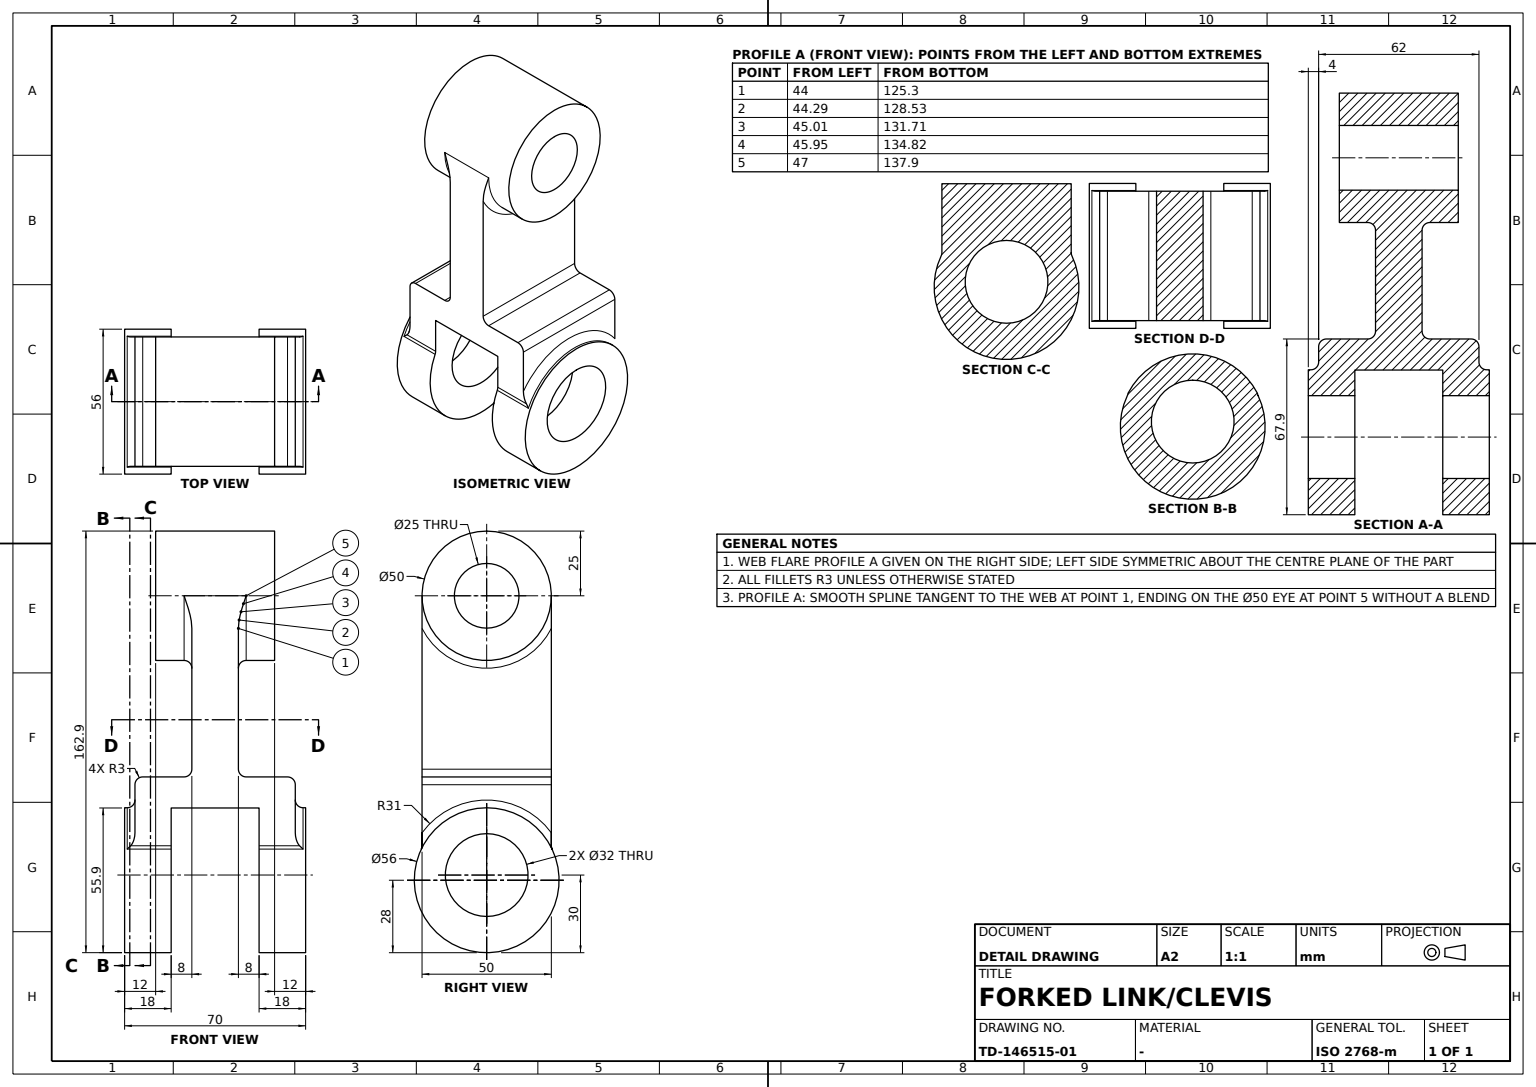
ISO-10303-21;
HEADER;
FILE_DESCRIPTION((''),'2;1');
FILE_NAME('','',(''),(''),'','','');
FILE_SCHEMA(('AUTOMOTIVE_DESIGN'));
ENDSEC;
DATA;
#1=APPLICATION_CONTEXT('');
#2=PRODUCT_CONTEXT('',#1,'mechanical');
#3=PRODUCT('','','',(#2));
#4=PRODUCT_DEFINITION_FORMATION('','',#3);
#5=PRODUCT_DEFINITION_CONTEXT('',#1,'design');
#6=PRODUCT_DEFINITION('','',#4,#5);
#7=PRODUCT_DEFINITION_SHAPE('','',#6);
#8=(LENGTH_UNIT()NAMED_UNIT(*)SI_UNIT(.MILLI.,.METRE.));
#9=(NAMED_UNIT(*)PLANE_ANGLE_UNIT()SI_UNIT($,.RADIAN.));
#10=(NAMED_UNIT(*)SI_UNIT($,.STERADIAN.)SOLID_ANGLE_UNIT());
#11=UNCERTAINTY_MEASURE_WITH_UNIT(LENGTH_MEASURE(0.005),#8,'distance_accuracy_value','');
#12=(GEOMETRIC_REPRESENTATION_CONTEXT(3)GLOBAL_UNCERTAINTY_ASSIGNED_CONTEXT((#11))GLOBAL_UNIT_ASSIGNED_CONTEXT((#8,#9,#10))REPRESENTATION_CONTEXT('',''));
#13=CARTESIAN_POINT('',(-25.,17.,-6.60046));
#14=VERTEX_POINT('',#13);
#15=CARTESIAN_POINT('',(-25.,32.652525,-6.600377));
#16=VERTEX_POINT('',#15);
#17=CARTESIAN_POINT('',(-25.,0.,-6.60046));
#18=DIRECTION('',(0.,-1.,0.));
#19=VECTOR('',#18,1000.);
#20=LINE('',#17,#19);
#21=EDGE_CURVE('',#14,#16,#20,.F.);
#22=ORIENTED_EDGE('',*,*,#21,.F.);
#23=CARTESIAN_POINT('',(-25.,17.,8.));
#24=VERTEX_POINT('',#23);
#25=CARTESIAN_POINT('',(-25.,17.,0.));
#26=DIRECTION('',(0.,0.,-1.));
#27=VECTOR('',#26,1000.);
#28=LINE('',#25,#27);
#29=EDGE_CURVE('',#24,#14,#28,.T.);
#30=ORIENTED_EDGE('',*,*,#29,.F.);
#31=CARTESIAN_POINT('',(-25.,-17.,8.));
#32=VERTEX_POINT('',#31);
#33=CARTESIAN_POINT('',(-25.,0.,8.));
#34=DIRECTION('',(0.,1.,0.));
#35=VECTOR('',#34,1000.);
#36=LINE('',#33,#35);
#37=EDGE_CURVE('',#32,#24,#36,.T.);
#38=ORIENTED_EDGE('',*,*,#37,.F.);
#39=CARTESIAN_POINT('',(-25.,-17.,-6.60046));
#40=VERTEX_POINT('',#39);
#41=CARTESIAN_POINT('',(-25.,-17.,0.));
#42=DIRECTION('',(0.,0.,1.));
#43=VECTOR('',#42,1000.);
#44=LINE('',#41,#43);
#45=EDGE_CURVE('',#40,#32,#44,.T.);
#46=ORIENTED_EDGE('',*,*,#45,.F.);
#47=CARTESIAN_POINT('',(-25.,-32.652602,-6.60046));
#48=VERTEX_POINT('',#47);
#49=EDGE_CURVE('',#40,#48,#20,.T.);
#50=ORIENTED_EDGE('',*,*,#49,.T.);
#51=CARTESIAN_POINT('',(-25.,-31.,-1.574292));
#52=VERTEX_POINT('',#51);
#53=CARTESIAN_POINT('',(-25.,-31.,-2.480429));
#54=CARTESIAN_POINT('',(-25.,-31.277064,-4.242952));
#55=CARTESIAN_POINT('',(-25.,-32.030566,-5.93486));
#56=B_SPLINE_CURVE_WITH_KNOTS('',3,(#51,#53,#54,#55,#47),.UNSPECIFIED.,.F.,.F.,(4,1,4),(0.,0.0026799,0.0053598),.UNSPECIFIED.);
#57=EDGE_CURVE('',#52,#48,#56,.T.);
#58=ORIENTED_EDGE('',*,*,#57,.F.);
#59=CARTESIAN_POINT('',(-25.,-31.,17.));
#60=VERTEX_POINT('',#59);
#61=CARTESIAN_POINT('',(-25.,-31.,0.));
#62=LINE('',#61,#27);
#63=EDGE_CURVE('',#60,#52,#62,.T.);
#64=ORIENTED_EDGE('',*,*,#63,.F.);
#65=CARTESIAN_POINT('',(-25.,-28.,20.));
#66=VERTEX_POINT('',#65);
#67=CARTESIAN_POINT('',(-25.,-28.,17.));
#68=DIRECTION('',(1.,0.,0.));
#69=AXIS2_PLACEMENT_3D('',#67,#68,#26);
#70=CIRCLE('',#69,3.);
#71=EDGE_CURVE('',#66,#60,#70,.T.);
#72=ORIENTED_EDGE('',*,*,#71,.F.);
#73=CARTESIAN_POINT('',(-25.,-12.,20.));
#74=VERTEX_POINT('',#73);
#75=CARTESIAN_POINT('',(-25.,0.,20.));
#76=LINE('',#75,#35);
#77=EDGE_CURVE('',#66,#74,#76,.T.);
#78=ORIENTED_EDGE('',*,*,#77,.T.);
#79=CARTESIAN_POINT('',(-25.,-9.,23.));
#80=VERTEX_POINT('',#79);
#81=CARTESIAN_POINT('',(-25.,-12.,23.));
#82=AXIS2_PLACEMENT_3D('',#81,#68,#26);
#83=CIRCLE('',#82,3.);
#84=EDGE_CURVE('',#74,#80,#83,.T.);
#85=ORIENTED_EDGE('',*,*,#84,.T.);
#86=CARTESIAN_POINT('',(-25.,-9.,77.39048));
#87=VERTEX_POINT('',#86);
#88=CARTESIAN_POINT('',(-25.,-9.,0.));
#89=LINE('',#88,#27);
#90=EDGE_CURVE('',#87,#80,#89,.T.);
#91=ORIENTED_EDGE('',*,*,#90,.F.);
#92=CARTESIAN_POINT('',(-25.,-12.,90.));
#93=VERTEX_POINT('',#92);
#94=CARTESIAN_POINT('',(-25.,-9.,79.576807));
#95=CARTESIAN_POINT('',(-25.,-9.867778,83.829787));
#96=CARTESIAN_POINT('',(-25.,-11.292251,87.956901));
#97=B_SPLINE_CURVE_WITH_KNOTS('',3,(#86,#94,#95,#96,#92),.UNSPECIFIED.,.F.,.F.,(4,1,4),(0.,0.006486638,0.012973277),.UNSPECIFIED.);
#98=EDGE_CURVE('',#87,#93,#97,.T.);
#99=ORIENTED_EDGE('',*,*,#98,.T.);
#100=CARTESIAN_POINT('',(-25.,12.,90.));
#101=VERTEX_POINT('',#100);
#102=CARTESIAN_POINT('',(-25.,0.,90.));
#103=LINE('',#102,#35);
#104=EDGE_CURVE('',#93,#101,#103,.T.);
#105=ORIENTED_EDGE('',*,*,#104,.T.);
#106=CARTESIAN_POINT('',(-25.,9.,77.39048));
#107=VERTEX_POINT('',#106);
#108=CARTESIAN_POINT('',(-25.,9.,79.576807));
#109=CARTESIAN_POINT('',(-25.,9.867778,83.829787));
#110=CARTESIAN_POINT('',(-25.,11.292251,87.956901));
#111=B_SPLINE_CURVE_WITH_KNOTS('',3,(#106,#108,#109,#110,#100),.UNSPECIFIED.,.F.,.F.,(4,1,4),(0.,0.006486638,0.012973277),.UNSPECIFIED.);
#112=EDGE_CURVE('',#107,#101,#111,.T.);
#113=ORIENTED_EDGE('',*,*,#112,.F.);
#114=CARTESIAN_POINT('',(-25.,9.,23.));
#115=VERTEX_POINT('',#114);
#116=CARTESIAN_POINT('',(-25.,9.,0.));
#117=LINE('',#116,#43);
#118=EDGE_CURVE('',#115,#107,#117,.T.);
#119=ORIENTED_EDGE('',*,*,#118,.F.);
#120=CARTESIAN_POINT('',(-25.,12.,20.));
#121=VERTEX_POINT('',#120);
#122=CARTESIAN_POINT('',(-25.,12.,23.));
#123=AXIS2_PLACEMENT_3D('',#122,#68,#26);
#124=CIRCLE('',#123,3.);
#125=EDGE_CURVE('',#115,#121,#124,.T.);
#126=ORIENTED_EDGE('',*,*,#125,.T.);
#127=CARTESIAN_POINT('',(-25.,28.,20.));
#128=VERTEX_POINT('',#127);
#129=EDGE_CURVE('',#121,#128,#76,.T.);
#130=ORIENTED_EDGE('',*,*,#129,.T.);
#131=CARTESIAN_POINT('',(-25.,31.,17.));
#132=VERTEX_POINT('',#131);
#133=CARTESIAN_POINT('',(-25.,28.,17.));
#134=AXIS2_PLACEMENT_3D('',#133,#68,#26);
#135=CIRCLE('',#134,3.);
#136=EDGE_CURVE('',#132,#128,#135,.T.);
#137=ORIENTED_EDGE('',*,*,#136,.F.);
#138=CARTESIAN_POINT('',(-25.,31.,-1.574292));
#139=VERTEX_POINT('',#138);
#140=CARTESIAN_POINT('',(-25.,31.,0.));
#141=LINE('',#140,#43);
#142=EDGE_CURVE('',#139,#132,#141,.T.);
#143=ORIENTED_EDGE('',*,*,#142,.F.);
#144=CARTESIAN_POINT('',(-25.,31.,-2.480411));
#145=CARTESIAN_POINT('',(-25.,31.277053,-4.2429));
#146=CARTESIAN_POINT('',(-25.,32.030524,-5.93477));
#147=B_SPLINE_CURVE_WITH_KNOTS('',3,(#138,#144,#145,#146,#15),.UNSPECIFIED.,.F.,.F.,(4,1,4),(0.,0.002679845,0.005359689),.UNSPECIFIED.);
#148=EDGE_CURVE('',#139,#16,#147,.T.);
#149=ORIENTED_EDGE('',*,*,#148,.T.);
#150=EDGE_LOOP('',(#22,#30,#38,#46,#50,#58,#64,#72,#78,#85,#91,#99,#105,#113,#119,#126,#130,#137,#143,#149));
#151=FACE_BOUND('',#150,.T.);
#152=CARTESIAN_POINT('',(-25.,0.,0.));
#153=AXIS2_PLACEMENT_3D('',#152,#68,#34);
#154=PLANE('',#153);
#155=ADVANCED_FACE('',(#151),#154,.F.);
#156=CARTESIAN_POINT('',(25.,9.,23.));
#157=VERTEX_POINT('',#156);
#158=CARTESIAN_POINT('',(25.,9.,77.39048));
#159=VERTEX_POINT('',#158);
#160=CARTESIAN_POINT('',(25.,9.,0.));
#161=LINE('',#160,#43);
#162=EDGE_CURVE('',#157,#159,#161,.T.);
#163=ORIENTED_EDGE('',*,*,#162,.F.);
#164=CARTESIAN_POINT('',(0.,9.,23.));
#165=VECTOR('',#68,1000.);
#166=LINE('',#164,#165);
#167=EDGE_CURVE('',#115,#157,#166,.T.);
#168=ORIENTED_EDGE('',*,*,#167,.F.);
#169=ORIENTED_EDGE('',*,*,#118,.T.);
#170=CARTESIAN_POINT('',(0.,9.,90.));
#171=AXIS2_PLACEMENT_3D('',#170,#34,#42);
#172=CIRCLE('',#171,28.);
#173=EDGE_CURVE('',#159,#107,#172,.T.);
#174=ORIENTED_EDGE('',*,*,#173,.F.);
#175=EDGE_LOOP('',(#163,#168,#169,#174));
#176=FACE_BOUND('',#175,.T.);
#177=CARTESIAN_POINT('',(0.,9.,20.));
#178=AXIS2_PLACEMENT_3D('',#177,#34,#42);
#179=PLANE('',#178);
#180=ADVANCED_FACE('',(#176),#179,.T.);
#181=CARTESIAN_POINT('',(0.,17.,-33.904594));
#182=VERTEX_POINT('',#181);
#183=CARTESIAN_POINT('',(0.,17.,-17.904594));
#184=AXIS2_PLACEMENT_3D('',#183,#18,#26);
#185=CIRCLE('',#184,16.);
#186=EDGE_CURVE('',#182,#182,#185,.T.);
#187=ORIENTED_EDGE('',*,*,#186,.T.);
#188=EDGE_LOOP('',(#187));
#189=FACE_BOUND('',#188,.T.);
#190=CARTESIAN_POINT('',(0.,35.,-1.904594));
#191=VERTEX_POINT('',#190);
#192=CARTESIAN_POINT('',(0.,35.,-17.904594));
#193=AXIS2_PLACEMENT_3D('',#192,#34,#42);
#194=CIRCLE('',#193,16.);
#195=EDGE_CURVE('',#191,#191,#194,.T.);
#196=ORIENTED_EDGE('',*,*,#195,.T.);
#197=EDGE_LOOP('',(#196));
#198=FACE_BOUND('',#197,.T.);
#199=CARTESIAN_POINT('',(0.,-0.66,-17.904594));
#200=DIRECTION('',(-1.,0.,0.));
#201=AXIS2_PLACEMENT_3D('',#199,#34,#200);
#202=CYLINDRICAL_SURFACE('',#201,16.);
#203=ADVANCED_FACE('',(#189,#198),#202,.F.);
#204=CARTESIAN_POINT('',(-25.290323,34.,-7.887957));
#205=VERTEX_POINT('',#204);
#206=CARTESIAN_POINT('',(25.290323,34.,-7.887957));
#207=VERTEX_POINT('',#206);
#208=CARTESIAN_POINT('',(0.,34.,-19.904594));
#209=AXIS2_PLACEMENT_3D('',#208,#34,#42);
#210=CIRCLE('',#209,28.);
#211=EDGE_CURVE('',#205,#207,#210,.T.);
#212=ORIENTED_EDGE('',*,*,#211,.F.);
#213=CARTESIAN_POINT('',(-25.104442,33.544266,-7.49675));
#214=CARTESIAN_POINT('',(-24.999987,33.086624,-7.064884));
#215=B_SPLINE_CURVE_WITH_KNOTS('',3,(#204,#213,#214,#15),.UNSPECIFIED.,.F.,.F.,(4,4),(-0.000010954,0.001875201),.UNSPECIFIED.);
#216=EDGE_CURVE('',#205,#16,#215,.T.);
#217=ORIENTED_EDGE('',*,*,#216,.T.);
#218=ORIENTED_EDGE('',*,*,#148,.F.);
#219=CARTESIAN_POINT('',(25.,31.,-1.574292));
#220=VERTEX_POINT('',#219);
#221=CARTESIAN_POINT('',(0.,31.,-19.904594));
#222=AXIS2_PLACEMENT_3D('',#221,#34,#42);
#223=CIRCLE('',#222,31.);
#224=EDGE_CURVE('',#139,#220,#223,.T.);
#225=ORIENTED_EDGE('',*,*,#224,.T.);
#226=CARTESIAN_POINT('',(25.,32.652525,-6.600377));
#227=VERTEX_POINT('',#226);
#228=CARTESIAN_POINT('',(25.,31.,-2.480411));
#229=CARTESIAN_POINT('',(25.,31.277053,-4.2429));
#230=CARTESIAN_POINT('',(25.,32.030524,-5.93477));
#231=B_SPLINE_CURVE_WITH_KNOTS('',3,(#219,#228,#229,#230,#226),.UNSPECIFIED.,.F.,.F.,(4,1,4),(0.,0.002679845,0.005359689),.UNSPECIFIED.);
#232=EDGE_CURVE('',#220,#227,#231,.T.);
#233=ORIENTED_EDGE('',*,*,#232,.T.);
#234=CARTESIAN_POINT('',(25.104442,33.544266,-7.49675));
#235=CARTESIAN_POINT('',(24.999987,33.086624,-7.064884));
#236=B_SPLINE_CURVE_WITH_KNOTS('',3,(#206,#234,#235,#226),.UNSPECIFIED.,.F.,.F.,(4,4),(-0.000010954,0.001875201),.UNSPECIFIED.);
#237=EDGE_CURVE('',#207,#227,#236,.T.);
#238=ORIENTED_EDGE('',*,*,#237,.F.);
#239=EDGE_LOOP('',(#212,#217,#218,#225,#233,#238));
#240=FACE_BOUND('',#239,.T.);
#241=DIRECTION('',(-0.613717662,0.,-0.789525574));
#242=AXIS2_PLACEMENT_3D('',#208,#34,#241);
#243=TOROIDAL_SURFACE('',#242,31.,3.);
#244=ADVANCED_FACE('',(#240),#243,.F.);
#245=CARTESIAN_POINT('',(25.,-31.,17.));
#246=VERTEX_POINT('',#245);
#247=CARTESIAN_POINT('',(25.,-31.,-1.574292));
#248=VERTEX_POINT('',#247);
#249=CARTESIAN_POINT('',(25.,-31.,0.));
#250=LINE('',#249,#27);
#251=EDGE_CURVE('',#246,#248,#250,.T.);
#252=ORIENTED_EDGE('',*,*,#251,.F.);
#253=CARTESIAN_POINT('',(0.,-31.,17.));
#254=LINE('',#253,#165);
#255=EDGE_CURVE('',#60,#246,#254,.T.);
#256=ORIENTED_EDGE('',*,*,#255,.F.);
#257=ORIENTED_EDGE('',*,*,#63,.T.);
#258=CARTESIAN_POINT('',(0.,-31.,-19.904594));
#259=AXIS2_PLACEMENT_3D('',#258,#18,#26);
#260=CIRCLE('',#259,31.);
#261=EDGE_CURVE('',#248,#52,#260,.T.);
#262=ORIENTED_EDGE('',*,*,#261,.F.);
#263=EDGE_LOOP('',(#252,#256,#257,#262));
#264=FACE_BOUND('',#263,.T.);
#265=CARTESIAN_POINT('',(0.,-31.,20.));
#266=AXIS2_PLACEMENT_3D('',#265,#18,#26);
#267=PLANE('',#266);
#268=ADVANCED_FACE('',(#264),#267,.T.);
#269=CARTESIAN_POINT('',(0.,23.,102.5));
#270=VERTEX_POINT('',#269);
#271=CARTESIAN_POINT('',(0.,23.,90.));
#272=AXIS2_PLACEMENT_3D('',#271,#34,#42);
#273=CIRCLE('',#272,12.5);
#274=EDGE_CURVE('',#270,#270,#273,.T.);
#275=ORIENTED_EDGE('',*,*,#274,.F.);
#276=EDGE_LOOP('',(#275));
#277=FACE_BOUND('',#276,.T.);
#278=CARTESIAN_POINT('',(0.,23.,115.));
#279=VERTEX_POINT('',#278);
#280=CIRCLE('',#272,25.);
#281=EDGE_CURVE('',#279,#279,#280,.T.);
#282=ORIENTED_EDGE('',*,*,#281,.T.);
#283=EDGE_LOOP('',(#282));
#284=FACE_BOUND('',#283,.T.);
#285=CARTESIAN_POINT('',(0.,23.,0.));
#286=AXIS2_PLACEMENT_3D('',#285,#34,#200);
#287=PLANE('',#286);
#288=ADVANCED_FACE('',(#277,#284),#287,.T.);
#289=CARTESIAN_POINT('',(0.,-35.,-1.904594));
#290=VERTEX_POINT('',#289);
#291=CARTESIAN_POINT('',(0.,-35.,-17.904594));
#292=AXIS2_PLACEMENT_3D('',#291,#34,#42);
#293=CIRCLE('',#292,16.);
#294=EDGE_CURVE('',#290,#290,#293,.T.);
#295=ORIENTED_EDGE('',*,*,#294,.T.);
#296=EDGE_LOOP('',(#295));
#297=FACE_BOUND('',#296,.T.);
#298=CARTESIAN_POINT('',(0.,-35.,8.095406));
#299=VERTEX_POINT('',#298);
#300=CARTESIAN_POINT('',(0.,-35.,-19.904594));
#301=AXIS2_PLACEMENT_3D('',#300,#34,#42);
#302=CIRCLE('',#301,28.);
#303=EDGE_CURVE('',#299,#299,#302,.T.);
#304=ORIENTED_EDGE('',*,*,#303,.F.);
#305=EDGE_LOOP('',(#304));
#306=FACE_BOUND('',#305,.T.);
#307=CARTESIAN_POINT('',(0.,-35.,0.));
#308=AXIS2_PLACEMENT_3D('',#307,#34,#200);
#309=PLANE('',#308);
#310=ADVANCED_FACE('',(#297,#306),#309,.F.);
#311=CARTESIAN_POINT('',(25.,-9.,23.));
#312=VERTEX_POINT('',#311);
#313=CARTESIAN_POINT('',(0.,-9.,23.));
#314=LINE('',#313,#165);
#315=EDGE_CURVE('',#80,#312,#314,.T.);
#316=ORIENTED_EDGE('',*,*,#315,.T.);
#317=CARTESIAN_POINT('',(25.,-9.,77.39048));
#318=VERTEX_POINT('',#317);
#319=CARTESIAN_POINT('',(25.,-9.,0.));
#320=LINE('',#319,#27);
#321=EDGE_CURVE('',#318,#312,#320,.T.);
#322=ORIENTED_EDGE('',*,*,#321,.F.);
#323=CARTESIAN_POINT('',(0.,-9.,90.));
#324=AXIS2_PLACEMENT_3D('',#323,#18,#26);
#325=CIRCLE('',#324,28.);
#326=EDGE_CURVE('',#87,#318,#325,.T.);
#327=ORIENTED_EDGE('',*,*,#326,.F.);
#328=ORIENTED_EDGE('',*,*,#90,.T.);
#329=EDGE_LOOP('',(#316,#322,#327,#328));
#330=FACE_BOUND('',#329,.T.);
#331=PLANE('',#324);
#332=ADVANCED_FACE('',(#330),#331,.T.);
#333=CARTESIAN_POINT('',(0.,-23.,115.));
#334=VERTEX_POINT('',#333);
#335=CARTESIAN_POINT('',(0.,-23.,90.));
#336=AXIS2_PLACEMENT_3D('',#335,#34,#42);
#337=CIRCLE('',#336,25.);
#338=EDGE_CURVE('',#334,#334,#337,.T.);
#339=ORIENTED_EDGE('',*,*,#338,.T.);
#340=EDGE_LOOP('',(#339));
#341=FACE_BOUND('',#340,.T.);
#342=ORIENTED_EDGE('',*,*,#281,.F.);
#343=EDGE_LOOP('',(#342));
#344=FACE_BOUND('',#343,.T.);
#345=CARTESIAN_POINT('',(25.,12.,90.));
#346=VERTEX_POINT('',#345);
#347=CARTESIAN_POINT('',(0.,12.,90.));
#348=AXIS2_PLACEMENT_3D('',#347,#34,#42);
#349=CIRCLE('',#348,25.);
#350=EDGE_CURVE('',#346,#101,#349,.T.);
#351=ORIENTED_EDGE('',*,*,#350,.T.);
#352=ORIENTED_EDGE('',*,*,#104,.F.);
#353=CARTESIAN_POINT('',(25.,-12.,90.));
#354=VERTEX_POINT('',#353);
#355=CARTESIAN_POINT('',(0.,-12.,90.));
#356=AXIS2_PLACEMENT_3D('',#355,#34,#42);
#357=CIRCLE('',#356,25.);
#358=EDGE_CURVE('',#93,#354,#357,.F.);
#359=ORIENTED_EDGE('',*,*,#358,.T.);
#360=CARTESIAN_POINT('',(25.,0.,90.));
#361=LINE('',#360,#35);
#362=EDGE_CURVE('',#354,#346,#361,.T.);
#363=ORIENTED_EDGE('',*,*,#362,.T.);
#364=EDGE_LOOP('',(#351,#352,#359,#363));
#365=FACE_BOUND('',#364,.T.);
#366=CARTESIAN_POINT('',(0.,0.,90.));
#367=AXIS2_PLACEMENT_3D('',#366,#34,#200);
#368=CYLINDRICAL_SURFACE('',#367,25.);
#369=ADVANCED_FACE('',(#341,#344,#365),#368,.T.);
#370=CARTESIAN_POINT('',(25.,-32.652602,-6.60046));
#371=VERTEX_POINT('',#370);
#372=CARTESIAN_POINT('',(25.,-31.,-2.480429));
#373=CARTESIAN_POINT('',(25.,-31.277064,-4.242952));
#374=CARTESIAN_POINT('',(25.,-32.030566,-5.93486));
#375=B_SPLINE_CURVE_WITH_KNOTS('',3,(#247,#372,#373,#374,#370),.UNSPECIFIED.,.F.,.F.,(4,1,4),(0.,0.0026799,0.0053598),.UNSPECIFIED.);
#376=EDGE_CURVE('',#248,#371,#375,.T.);
#377=ORIENTED_EDGE('',*,*,#376,.F.);
#378=ORIENTED_EDGE('',*,*,#261,.T.);
#379=ORIENTED_EDGE('',*,*,#57,.T.);
#380=CARTESIAN_POINT('',(-25.290323,-34.,-7.887957));
#381=VERTEX_POINT('',#380);
#382=CARTESIAN_POINT('',(-25.104453,-33.544293,-7.496773));
#383=CARTESIAN_POINT('',(-25.,-33.086677,-7.064935));
#384=B_SPLINE_CURVE_WITH_KNOTS('',3,(#380,#382,#383,#47),.UNSPECIFIED.,.F.,.F.,(4,4),(-0.000010954,0.00187509),.UNSPECIFIED.);
#385=EDGE_CURVE('',#381,#48,#384,.T.);
#386=ORIENTED_EDGE('',*,*,#385,.F.);
#387=CARTESIAN_POINT('',(25.290323,-34.,-7.887957));
#388=VERTEX_POINT('',#387);
#389=CARTESIAN_POINT('',(0.,-34.,-19.904594));
#390=AXIS2_PLACEMENT_3D('',#389,#34,#42);
#391=CIRCLE('',#390,28.);
#392=EDGE_CURVE('',#388,#381,#391,.F.);
#393=ORIENTED_EDGE('',*,*,#392,.F.);
#394=CARTESIAN_POINT('',(25.104453,-33.544293,-7.496773));
#395=CARTESIAN_POINT('',(25.,-33.086677,-7.064935));
#396=B_SPLINE_CURVE_WITH_KNOTS('',3,(#387,#394,#395,#370),.UNSPECIFIED.,.F.,.F.,(4,4),(-0.000010954,0.00187509),.UNSPECIFIED.);
#397=EDGE_CURVE('',#388,#371,#396,.T.);
#398=ORIENTED_EDGE('',*,*,#397,.T.);
#399=EDGE_LOOP('',(#377,#378,#379,#386,#393,#398));
#400=FACE_BOUND('',#399,.T.);
#401=DIRECTION('',(0.547489236,0.,-0.836812725));
#402=AXIS2_PLACEMENT_3D('',#389,#18,#401);
#403=TOROIDAL_SURFACE('',#402,31.,3.);
#404=ADVANCED_FACE('',(#400),#403,.F.);
#405=CARTESIAN_POINT('',(25.,12.,20.));
#406=VERTEX_POINT('',#405);
#407=CARTESIAN_POINT('',(0.,12.,20.));
#408=LINE('',#407,#165);
#409=EDGE_CURVE('',#121,#406,#408,.T.);
#410=ORIENTED_EDGE('',*,*,#409,.F.);
#411=ORIENTED_EDGE('',*,*,#125,.F.);
#412=ORIENTED_EDGE('',*,*,#167,.T.);
#413=CARTESIAN_POINT('',(25.,12.,23.));
#414=AXIS2_PLACEMENT_3D('',#413,#68,#26);
#415=CIRCLE('',#414,3.);
#416=EDGE_CURVE('',#157,#406,#415,.T.);
#417=ORIENTED_EDGE('',*,*,#416,.T.);
#418=EDGE_LOOP('',(#410,#411,#412,#417));
#419=FACE_BOUND('',#418,.T.);
#420=CARTESIAN_POINT('',(0.,12.,23.));
#421=AXIS2_PLACEMENT_3D('',#420,#68,#18);
#422=CYLINDRICAL_SURFACE('',#421,3.);
#423=ADVANCED_FACE('',(#419),#422,.F.);
#424=ORIENTED_EDGE('',*,*,#294,.F.);
#425=EDGE_LOOP('',(#424));
#426=FACE_BOUND('',#425,.T.);
#427=CARTESIAN_POINT('',(0.,-17.,-1.904594));
#428=VERTEX_POINT('',#427);
#429=CARTESIAN_POINT('',(0.,-17.,-17.904594));
#430=AXIS2_PLACEMENT_3D('',#429,#34,#42);
#431=CIRCLE('',#430,16.);
#432=EDGE_CURVE('',#428,#428,#431,.T.);
#433=ORIENTED_EDGE('',*,*,#432,.T.);
#434=EDGE_LOOP('',(#433));
#435=FACE_BOUND('',#434,.T.);
#436=ADVANCED_FACE('',(#426,#435),#202,.F.);
#437=ORIENTED_EDGE('',*,*,#216,.F.);
#438=CARTESIAN_POINT('',(-25.290323,17.,-7.887957));
#439=VERTEX_POINT('',#438);
#440=CARTESIAN_POINT('',(-25.290323,25.5,-7.887957));
#441=LINE('',#440,#19);
#442=EDGE_CURVE('',#439,#205,#441,.F.);
#443=ORIENTED_EDGE('',*,*,#442,.F.);
#444=CARTESIAN_POINT('',(-28.,17.,-6.60046));
#445=AXIS2_PLACEMENT_3D('',#444,#18,#26);
#446=CIRCLE('',#445,3.);
#447=EDGE_CURVE('',#439,#14,#446,.T.);
#448=ORIENTED_EDGE('',*,*,#447,.T.);
#449=ORIENTED_EDGE('',*,*,#21,.T.);
#450=EDGE_LOOP('',(#437,#443,#448,#449));
#451=FACE_BOUND('',#450,.T.);
#452=CARTESIAN_POINT('',(-28.,0.,-6.60046));
#453=AXIS2_PLACEMENT_3D('',#452,#18,#68);
#454=CYLINDRICAL_SURFACE('',#453,3.);
#455=ADVANCED_FACE('',(#451),#454,.F.);
#456=CARTESIAN_POINT('',(25.,9.,79.576807));
#457=CARTESIAN_POINT('',(25.,9.867778,83.829787));
#458=CARTESIAN_POINT('',(25.,11.292251,87.956901));
#459=B_SPLINE_CURVE_WITH_KNOTS('',3,(#158,#456,#457,#458,#345),.UNSPECIFIED.,.F.,.F.,(4,1,4),(0.,0.006486638,0.012973277),.UNSPECIFIED.);
#460=EDGE_CURVE('',#159,#346,#459,.T.);
#461=ORIENTED_EDGE('',*,*,#460,.F.);
#462=ORIENTED_EDGE('',*,*,#173,.T.);
#463=ORIENTED_EDGE('',*,*,#112,.T.);
#464=ORIENTED_EDGE('',*,*,#350,.F.);
#465=EDGE_LOOP('',(#461,#462,#463,#464));
#466=FACE_BOUND('',#465,.T.);
#467=DIRECTION('',(0.641258302,0.,0.767325087));
#468=AXIS2_PLACEMENT_3D('',#347,#34,#467);
#469=TOROIDAL_SURFACE('',#468,28.,3.);
#470=ADVANCED_FACE('',(#466),#469,.F.);
#471=CARTESIAN_POINT('',(25.,17.,8.));
#472=VERTEX_POINT('',#471);
#473=CARTESIAN_POINT('',(25.,17.,-6.60046));
#474=VERTEX_POINT('',#473);
#475=CARTESIAN_POINT('',(25.,17.,0.));
#476=LINE('',#475,#27);
#477=EDGE_CURVE('',#472,#474,#476,.T.);
#478=ORIENTED_EDGE('',*,*,#477,.T.);
#479=CARTESIAN_POINT('',(25.,0.,-6.60046));
#480=LINE('',#479,#19);
#481=EDGE_CURVE('',#474,#227,#480,.F.);
#482=ORIENTED_EDGE('',*,*,#481,.T.);
#483=ORIENTED_EDGE('',*,*,#232,.F.);
#484=CARTESIAN_POINT('',(25.,31.,17.));
#485=VERTEX_POINT('',#484);
#486=CARTESIAN_POINT('',(25.,31.,0.));
#487=LINE('',#486,#43);
#488=EDGE_CURVE('',#220,#485,#487,.T.);
#489=ORIENTED_EDGE('',*,*,#488,.T.);
#490=CARTESIAN_POINT('',(25.,28.,20.));
#491=VERTEX_POINT('',#490);
#492=CARTESIAN_POINT('',(25.,28.,17.));
#493=AXIS2_PLACEMENT_3D('',#492,#68,#26);
#494=CIRCLE('',#493,3.);
#495=EDGE_CURVE('',#485,#491,#494,.T.);
#496=ORIENTED_EDGE('',*,*,#495,.T.);
#497=CARTESIAN_POINT('',(25.,0.,20.));
#498=LINE('',#497,#35);
#499=EDGE_CURVE('',#406,#491,#498,.T.);
#500=ORIENTED_EDGE('',*,*,#499,.F.);
#501=ORIENTED_EDGE('',*,*,#416,.F.);
#502=ORIENTED_EDGE('',*,*,#162,.T.);
#503=ORIENTED_EDGE('',*,*,#460,.T.);
#504=ORIENTED_EDGE('',*,*,#362,.F.);
#505=CARTESIAN_POINT('',(25.,-9.,79.576807));
#506=CARTESIAN_POINT('',(25.,-9.867778,83.829787));
#507=CARTESIAN_POINT('',(25.,-11.292251,87.956901));
#508=B_SPLINE_CURVE_WITH_KNOTS('',3,(#317,#505,#506,#507,#353),.UNSPECIFIED.,.F.,.F.,(4,1,4),(0.,0.006486638,0.012973277),.UNSPECIFIED.);
#509=EDGE_CURVE('',#318,#354,#508,.T.);
#510=ORIENTED_EDGE('',*,*,#509,.F.);
#511=ORIENTED_EDGE('',*,*,#321,.T.);
#512=CARTESIAN_POINT('',(25.,-12.,20.));
#513=VERTEX_POINT('',#512);
#514=CARTESIAN_POINT('',(25.,-12.,23.));
#515=AXIS2_PLACEMENT_3D('',#514,#68,#26);
#516=CIRCLE('',#515,3.);
#517=EDGE_CURVE('',#513,#312,#516,.T.);
#518=ORIENTED_EDGE('',*,*,#517,.F.);
#519=CARTESIAN_POINT('',(25.,-28.,20.));
#520=VERTEX_POINT('',#519);
#521=EDGE_CURVE('',#520,#513,#498,.T.);
#522=ORIENTED_EDGE('',*,*,#521,.F.);
#523=CARTESIAN_POINT('',(25.,-28.,17.));
#524=AXIS2_PLACEMENT_3D('',#523,#68,#26);
#525=CIRCLE('',#524,3.);
#526=EDGE_CURVE('',#520,#246,#525,.T.);
#527=ORIENTED_EDGE('',*,*,#526,.T.);
#528=ORIENTED_EDGE('',*,*,#251,.T.);
#529=ORIENTED_EDGE('',*,*,#376,.T.);
#530=CARTESIAN_POINT('',(25.,-17.,-6.60046));
#531=VERTEX_POINT('',#530);
#532=EDGE_CURVE('',#531,#371,#480,.T.);
#533=ORIENTED_EDGE('',*,*,#532,.F.);
#534=CARTESIAN_POINT('',(25.,-17.,8.));
#535=VERTEX_POINT('',#534);
#536=CARTESIAN_POINT('',(25.,-17.,0.));
#537=LINE('',#536,#43);
#538=EDGE_CURVE('',#531,#535,#537,.T.);
#539=ORIENTED_EDGE('',*,*,#538,.T.);
#540=CARTESIAN_POINT('',(25.,0.,8.));
#541=LINE('',#540,#35);
#542=EDGE_CURVE('',#535,#472,#541,.T.);
#543=ORIENTED_EDGE('',*,*,#542,.T.);
#544=EDGE_LOOP('',(#478,#482,#483,#489,#496,#500,#501,#502,#503,#504,#510,#511,#518,#522,#527,#528,#529,#533,#539,#543));
#545=FACE_BOUND('',#544,.T.);
#546=CARTESIAN_POINT('',(25.,0.,0.));
#547=AXIS2_PLACEMENT_3D('',#546,#68,#34);
#548=PLANE('',#547);
#549=ADVANCED_FACE('',(#545),#548,.T.);
#550=CARTESIAN_POINT('',(0.,17.,8.));
#551=LINE('',#550,#165);
#552=EDGE_CURVE('',#24,#472,#551,.T.);
#553=ORIENTED_EDGE('',*,*,#552,.T.);
#554=ORIENTED_EDGE('',*,*,#542,.F.);
#555=CARTESIAN_POINT('',(0.,-17.,8.));
#556=LINE('',#555,#165);
#557=EDGE_CURVE('',#32,#535,#556,.T.);
#558=ORIENTED_EDGE('',*,*,#557,.F.);
#559=ORIENTED_EDGE('',*,*,#37,.T.);
#560=EDGE_LOOP('',(#553,#554,#558,#559));
#561=FACE_BOUND('',#560,.T.);
#562=AXIS2_PLACEMENT_3D('',#555,#26,#34);
#563=PLANE('',#562);
#564=ADVANCED_FACE('',(#561),#563,.T.);
#565=ORIENTED_EDGE('',*,*,#481,.F.);
#566=CARTESIAN_POINT('',(25.290323,17.,-7.887957));
#567=VERTEX_POINT('',#566);
#568=CARTESIAN_POINT('',(28.,17.,-6.60046));
#569=AXIS2_PLACEMENT_3D('',#568,#18,#26);
#570=CIRCLE('',#569,3.);
#571=EDGE_CURVE('',#474,#567,#570,.T.);
#572=ORIENTED_EDGE('',*,*,#571,.T.);
#573=CARTESIAN_POINT('',(25.290323,25.5,-7.887957));
#574=LINE('',#573,#35);
#575=EDGE_CURVE('',#567,#207,#574,.T.);
#576=ORIENTED_EDGE('',*,*,#575,.T.);
#577=ORIENTED_EDGE('',*,*,#237,.T.);
#578=EDGE_LOOP('',(#565,#572,#576,#577));
#579=FACE_BOUND('',#578,.T.);
#580=CARTESIAN_POINT('',(28.,0.,-6.60046));
#581=AXIS2_PLACEMENT_3D('',#580,#18,#200);
#582=CYLINDRICAL_SURFACE('',#581,3.);
#583=ADVANCED_FACE('',(#579),#582,.F.);
#584=CARTESIAN_POINT('',(0.,-28.,20.));
#585=LINE('',#584,#165);
#586=EDGE_CURVE('',#66,#520,#585,.T.);
#587=ORIENTED_EDGE('',*,*,#586,.F.);
#588=ORIENTED_EDGE('',*,*,#71,.T.);
#589=ORIENTED_EDGE('',*,*,#255,.T.);
#590=ORIENTED_EDGE('',*,*,#526,.F.);
#591=EDGE_LOOP('',(#587,#588,#589,#590));
#592=FACE_BOUND('',#591,.T.);
#593=CARTESIAN_POINT('',(0.,-28.,17.));
#594=AXIS2_PLACEMENT_3D('',#593,#68,#18);
#595=CYLINDRICAL_SURFACE('',#594,3.);
#596=ADVANCED_FACE('',(#592),#595,.T.);
#597=ORIENTED_EDGE('',*,*,#274,.T.);
#598=EDGE_LOOP('',(#597));
#599=FACE_BOUND('',#598,.T.);
#600=CARTESIAN_POINT('',(0.,-23.,102.5));
#601=VERTEX_POINT('',#600);
#602=CIRCLE('',#336,12.5);
#603=EDGE_CURVE('',#601,#601,#602,.T.);
#604=ORIENTED_EDGE('',*,*,#603,.F.);
#605=EDGE_LOOP('',(#604));
#606=FACE_BOUND('',#605,.T.);
#607=CARTESIAN_POINT('',(0.,-6.66,90.));
#608=AXIS2_PLACEMENT_3D('',#607,#34,#200);
#609=CYLINDRICAL_SURFACE('',#608,12.5);
#610=ADVANCED_FACE('',(#599,#606),#609,.F.);
#611=ORIENTED_EDGE('',*,*,#409,.T.);
#612=ORIENTED_EDGE('',*,*,#499,.T.);
#613=CARTESIAN_POINT('',(0.,28.,20.));
#614=LINE('',#613,#165);
#615=EDGE_CURVE('',#128,#491,#614,.T.);
#616=ORIENTED_EDGE('',*,*,#615,.F.);
#617=ORIENTED_EDGE('',*,*,#129,.F.);
#618=EDGE_LOOP('',(#611,#612,#616,#617));
#619=FACE_BOUND('',#618,.T.);
#620=AXIS2_PLACEMENT_3D('',#177,#26,#34);
#621=PLANE('',#620);
#622=ADVANCED_FACE('',(#619),#621,.F.);
#623=ORIENTED_EDGE('',*,*,#432,.F.);
#624=EDGE_LOOP('',(#623));
#625=FACE_BOUND('',#624,.T.);
#626=ORIENTED_EDGE('',*,*,#45,.T.);
#627=ORIENTED_EDGE('',*,*,#557,.T.);
#628=ORIENTED_EDGE('',*,*,#538,.F.);
#629=CARTESIAN_POINT('',(25.290323,-17.,-7.887957));
#630=VERTEX_POINT('',#629);
#631=CARTESIAN_POINT('',(28.,-17.,-6.60046));
#632=AXIS2_PLACEMENT_3D('',#631,#34,#42);
#633=CIRCLE('',#632,3.);
#634=EDGE_CURVE('',#630,#531,#633,.T.);
#635=ORIENTED_EDGE('',*,*,#634,.F.);
#636=CARTESIAN_POINT('',(-25.290323,-17.,-7.887957));
#637=VERTEX_POINT('',#636);
#638=CARTESIAN_POINT('',(0.,-17.,-19.904594));
#639=AXIS2_PLACEMENT_3D('',#638,#34,#42);
#640=CIRCLE('',#639,28.);
#641=EDGE_CURVE('',#630,#637,#640,.T.);
#642=ORIENTED_EDGE('',*,*,#641,.T.);
#643=CARTESIAN_POINT('',(-28.,-17.,-6.60046));
#644=AXIS2_PLACEMENT_3D('',#643,#34,#42);
#645=CIRCLE('',#644,3.);
#646=EDGE_CURVE('',#40,#637,#645,.T.);
#647=ORIENTED_EDGE('',*,*,#646,.F.);
#648=EDGE_LOOP('',(#626,#627,#628,#635,#642,#647));
#649=FACE_BOUND('',#648,.T.);
#650=CARTESIAN_POINT('',(0.,-17.,-20.));
#651=AXIS2_PLACEMENT_3D('',#650,#34,#42);
#652=PLANE('',#651);
#653=ADVANCED_FACE('',(#625,#649),#652,.T.);
#654=ORIENTED_EDGE('',*,*,#603,.T.);
#655=EDGE_LOOP('',(#654));
#656=FACE_BOUND('',#655,.T.);
#657=ORIENTED_EDGE('',*,*,#338,.F.);
#658=EDGE_LOOP('',(#657));
#659=FACE_BOUND('',#658,.T.);
#660=CARTESIAN_POINT('',(0.,-23.,0.));
#661=AXIS2_PLACEMENT_3D('',#660,#34,#200);
#662=PLANE('',#661);
#663=ADVANCED_FACE('',(#656,#659),#662,.F.);
#664=ORIENTED_EDGE('',*,*,#326,.T.);
#665=ORIENTED_EDGE('',*,*,#509,.T.);
#666=ORIENTED_EDGE('',*,*,#358,.F.);
#667=ORIENTED_EDGE('',*,*,#98,.F.);
#668=EDGE_LOOP('',(#664,#665,#666,#667));
#669=FACE_BOUND('',#668,.T.);
#670=DIRECTION('',(-0.766152877,0.,0.642658361));
#671=AXIS2_PLACEMENT_3D('',#355,#18,#670);
#672=TOROIDAL_SURFACE('',#671,28.,3.);
#673=ADVANCED_FACE('',(#669),#672,.F.);
#674=ORIENTED_EDGE('',*,*,#575,.F.);
#675=CARTESIAN_POINT('',(0.,17.,-19.904594));
#676=AXIS2_PLACEMENT_3D('',#675,#18,#26);
#677=CIRCLE('',#676,28.);
#678=EDGE_CURVE('',#567,#439,#677,.F.);
#679=ORIENTED_EDGE('',*,*,#678,.T.);
#680=ORIENTED_EDGE('',*,*,#442,.T.);
#681=ORIENTED_EDGE('',*,*,#211,.T.);
#682=EDGE_LOOP('',(#674,#679,#680,#681));
#683=FACE_BOUND('',#682,.T.);
#684=CARTESIAN_POINT('',(0.,35.,8.095406));
#685=VERTEX_POINT('',#684);
#686=CARTESIAN_POINT('',(0.,35.,-19.904594));
#687=AXIS2_PLACEMENT_3D('',#686,#34,#42);
#688=CIRCLE('',#687,28.);
#689=EDGE_CURVE('',#685,#685,#688,.T.);
#690=ORIENTED_EDGE('',*,*,#689,.F.);
#691=EDGE_LOOP('',(#690));
#692=FACE_BOUND('',#691,.T.);
#693=CARTESIAN_POINT('',(0.,-26.,-19.904594));
#694=AXIS2_PLACEMENT_3D('',#693,#34,#200);
#695=CYLINDRICAL_SURFACE('',#694,28.);
#696=ADVANCED_FACE('',(#683,#692),#695,.T.);
#697=ORIENTED_EDGE('',*,*,#303,.T.);
#698=EDGE_LOOP('',(#697));
#699=FACE_BOUND('',#698,.T.);
#700=CARTESIAN_POINT('',(25.290323,-25.5,-7.887957));
#701=LINE('',#700,#19);
#702=EDGE_CURVE('',#630,#388,#701,.T.);
#703=ORIENTED_EDGE('',*,*,#702,.T.);
#704=ORIENTED_EDGE('',*,*,#392,.T.);
#705=CARTESIAN_POINT('',(-25.290323,-25.5,-7.887957));
#706=LINE('',#705,#35);
#707=EDGE_CURVE('',#637,#381,#706,.F.);
#708=ORIENTED_EDGE('',*,*,#707,.F.);
#709=ORIENTED_EDGE('',*,*,#641,.F.);
#710=EDGE_LOOP('',(#703,#704,#708,#709));
#711=FACE_BOUND('',#710,.T.);
#712=ADVANCED_FACE('',(#699,#711),#695,.T.);
#713=ORIENTED_EDGE('',*,*,#77,.F.);
#714=ORIENTED_EDGE('',*,*,#586,.T.);
#715=ORIENTED_EDGE('',*,*,#521,.T.);
#716=CARTESIAN_POINT('',(0.,-12.,20.));
#717=LINE('',#716,#165);
#718=EDGE_CURVE('',#74,#513,#717,.T.);
#719=ORIENTED_EDGE('',*,*,#718,.F.);
#720=EDGE_LOOP('',(#713,#714,#715,#719));
#721=FACE_BOUND('',#720,.T.);
#722=ADVANCED_FACE('',(#721),#621,.F.);
#723=ORIENTED_EDGE('',*,*,#689,.T.);
#724=EDGE_LOOP('',(#723));
#725=FACE_BOUND('',#724,.T.);
#726=ORIENTED_EDGE('',*,*,#195,.F.);
#727=EDGE_LOOP('',(#726));
#728=FACE_BOUND('',#727,.T.);
#729=CARTESIAN_POINT('',(0.,35.,0.));
#730=AXIS2_PLACEMENT_3D('',#729,#34,#200);
#731=PLANE('',#730);
#732=ADVANCED_FACE('',(#725,#728),#731,.T.);
#733=ORIENTED_EDGE('',*,*,#634,.T.);
#734=ORIENTED_EDGE('',*,*,#532,.T.);
#735=ORIENTED_EDGE('',*,*,#397,.F.);
#736=ORIENTED_EDGE('',*,*,#702,.F.);
#737=EDGE_LOOP('',(#733,#734,#735,#736));
#738=FACE_BOUND('',#737,.T.);
#739=ADVANCED_FACE('',(#738),#582,.F.);
#740=ORIENTED_EDGE('',*,*,#707,.T.);
#741=ORIENTED_EDGE('',*,*,#385,.T.);
#742=ORIENTED_EDGE('',*,*,#49,.F.);
#743=ORIENTED_EDGE('',*,*,#646,.T.);
#744=EDGE_LOOP('',(#740,#741,#742,#743));
#745=FACE_BOUND('',#744,.T.);
#746=ADVANCED_FACE('',(#745),#454,.F.);
#747=ORIENTED_EDGE('',*,*,#678,.F.);
#748=ORIENTED_EDGE('',*,*,#571,.F.);
#749=ORIENTED_EDGE('',*,*,#477,.F.);
#750=ORIENTED_EDGE('',*,*,#552,.F.);
#751=ORIENTED_EDGE('',*,*,#29,.T.);
#752=ORIENTED_EDGE('',*,*,#447,.F.);
#753=EDGE_LOOP('',(#747,#748,#749,#750,#751,#752));
#754=FACE_BOUND('',#753,.T.);
#755=ORIENTED_EDGE('',*,*,#186,.F.);
#756=EDGE_LOOP('',(#755));
#757=FACE_BOUND('',#756,.T.);
#758=AXIS2_PLACEMENT_3D('',#550,#18,#26);
#759=PLANE('',#758);
#760=ADVANCED_FACE('',(#754,#757),#759,.T.);
#761=ORIENTED_EDGE('',*,*,#615,.T.);
#762=ORIENTED_EDGE('',*,*,#495,.F.);
#763=CARTESIAN_POINT('',(0.,31.,17.));
#764=LINE('',#763,#165);
#765=EDGE_CURVE('',#132,#485,#764,.T.);
#766=ORIENTED_EDGE('',*,*,#765,.F.);
#767=ORIENTED_EDGE('',*,*,#136,.T.);
#768=EDGE_LOOP('',(#761,#762,#766,#767));
#769=FACE_BOUND('',#768,.T.);
#770=CARTESIAN_POINT('',(0.,28.,17.));
#771=AXIS2_PLACEMENT_3D('',#770,#68,#42);
#772=CYLINDRICAL_SURFACE('',#771,3.);
#773=ADVANCED_FACE('',(#769),#772,.T.);
#774=ORIENTED_EDGE('',*,*,#142,.T.);
#775=ORIENTED_EDGE('',*,*,#765,.T.);
#776=ORIENTED_EDGE('',*,*,#488,.F.);
#777=ORIENTED_EDGE('',*,*,#224,.F.);
#778=EDGE_LOOP('',(#774,#775,#776,#777));
#779=FACE_BOUND('',#778,.T.);
#780=CARTESIAN_POINT('',(0.,31.,-20.));
#781=AXIS2_PLACEMENT_3D('',#780,#34,#42);
#782=PLANE('',#781);
#783=ADVANCED_FACE('',(#779),#782,.T.);
#784=ORIENTED_EDGE('',*,*,#315,.F.);
#785=ORIENTED_EDGE('',*,*,#84,.F.);
#786=ORIENTED_EDGE('',*,*,#718,.T.);
#787=ORIENTED_EDGE('',*,*,#517,.T.);
#788=EDGE_LOOP('',(#784,#785,#786,#787));
#789=FACE_BOUND('',#788,.T.);
#790=CARTESIAN_POINT('',(0.,-12.,23.));
#791=AXIS2_PLACEMENT_3D('',#790,#68,#26);
#792=CYLINDRICAL_SURFACE('',#791,3.);
#793=ADVANCED_FACE('',(#789),#792,.F.);
#794=CLOSED_SHELL('',(#155,#180,#203,#244,#268,#288,#310,#332,#369,#404,#423,#436,#455,#470,#549,#564,#583,#596,#610,#622,#653,#663,#673,#696,#712,#722,#732,#739,#746,#760,#773,#783,#793));
#795=MANIFOLD_SOLID_BREP('',#794);
#796=ADVANCED_BREP_SHAPE_REPRESENTATION('',(#795),#12);
#797=SHAPE_DEFINITION_REPRESENTATION(#7,#796);
ENDSEC;
END-ISO-10303-21;
